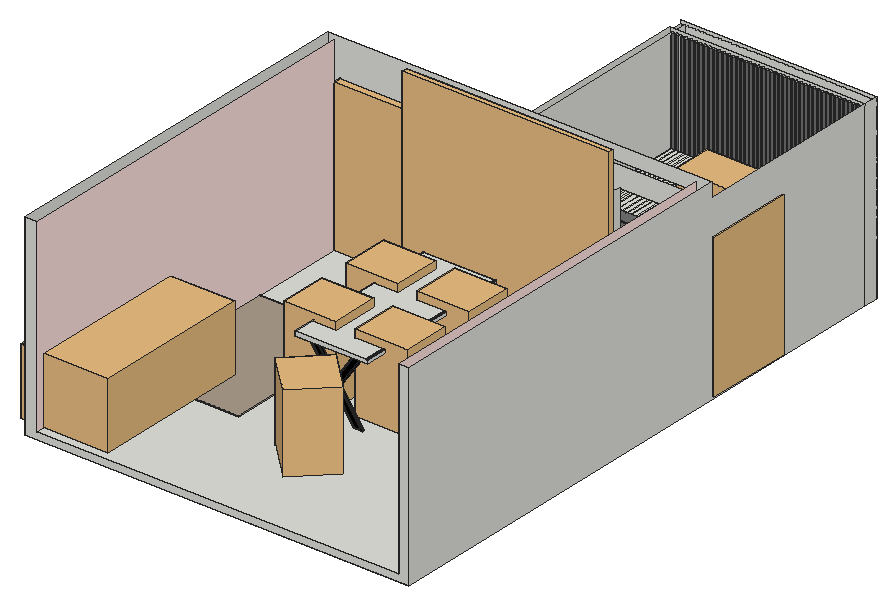
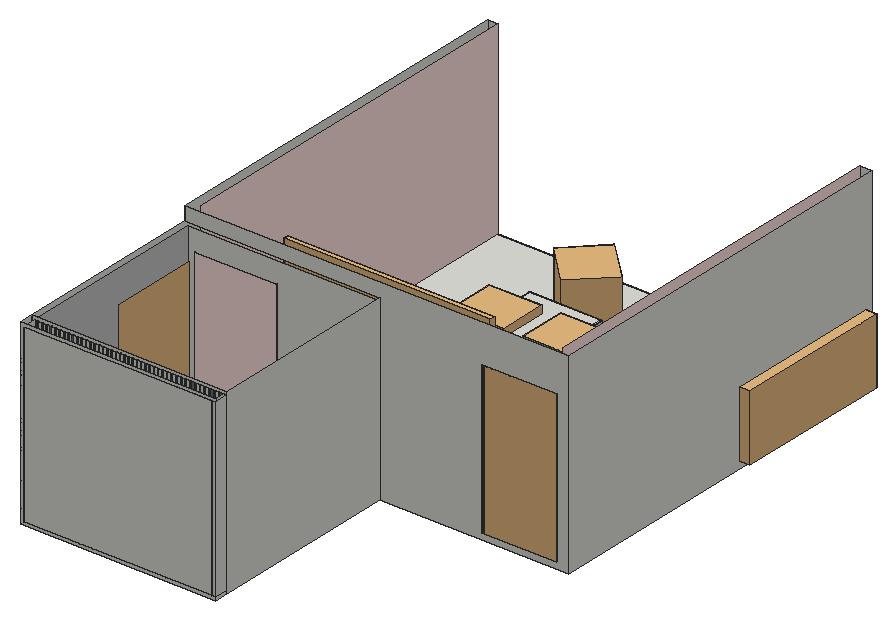
# SketchUp Ruby script. Lengths in inches.
U = 1.inch
M = Sketchup.active_model
def pt(a) = Geom::Point3d.new(a.map { |v| v * U })
def face(e, loops, mat)
  f = e.add_face(loops[0].map { |a| pt(a) })
  loops[1..].each { |l| e.add_face(l.map { |a| pt(a) }).erase! }
  f.material = f.back_material = mat if mat
  f
end
# faces: each face lists its corners as indices into pts; further lists are holes
def faces(e, pts, list, mat = nil) = list.each { |f| face(e, (f[0].is_a?(Array) ? f : [f]).map { |l| l.map { |i| pts[i] } }, mat) }
# xy, xz, yz: faces in a plane at the given z, y or x. An outline is a flat list of corners, or four numbers for a rectangle; further outlines are holes
def ring(l) = l.size == 4 ? [[l[0], l[1]], [l[2], l[1]], [l[2], l[3]], [l[0], l[3]]] : l.each_slice(2).to_a
def flat(e, list, mat, &to3) = list.each { |f| face(e, (f[0].is_a?(Array) ? f : [f]).map { |l| ring(l).map { |u, v| to3.(u, v) } }, mat) }
def xy(e, z, list, mat = nil) = flat(e, list, mat) { |x, y| [x, y, z] }
def xz(e, y, list, mat = nil) = flat(e, list, mat) { |x, z| [x, y, z] }
def yz(e, x, list, mat = nil) = flat(e, list, mat) { |y, z| [x, y, z] }
def lines(e, pts, list) = list.each { |a, b| e.add_line(pt(pts[a]), pt(pts[b])) }
# prism: a flat outline (further loops are holes) pulled along v
def prism(e, loops, v, mat = nil)
  f = face(e, loops, mat); d = Geom::Vector3d.new(v.map { |x| x * U })
  f.pushpull(f.normal.samedirection?(d) ? d.length : -d.length)
end
def box(e, o, s, mat = nil) = prism(e, [[o, [o[0] + s[0], o[1], o[2]], [o[0] + s[0], o[1] + s[1], o[2]], [o[0], o[1] + s[1], o[2]]]], [0, 0, s[2]], mat)
def at(x, y, z, deg = 0) = Geom::Transformation.translation(pt([x, y, z])) * Geom::Transformation.rotation(ORIGIN, Z_AXIS, deg.degrees)
def axes(o, x, y, z) = Geom::Transformation.new([*x, 0, *y, 0, *z, 0, *pt(o).to_a, 1])
def part(name) = M.definitions.add(name)
# library, detail: a bought-in or finely detailed component or shape, given as its bounding box
def library(name, o, s) = part(name).tap { |d| box(d.entities, o, s) }
def detail(e, o, s) = box(e.add_group.entities, o, s)
def put(e, d, t, mat = nil) = e.add_instance(d, t).tap { |i| i.material = mat if mat }
def group(e, t, mat = nil) = e.add_group.tap { |g| g.transformation = t; g.material = mat if mat }.entities
root = M.entities
M.materials.add("[0005_LightPink]").color = [255, 182, 193]
M.materials["[0005_LightPink]"].alpha = 0.48
M.materials.add("[0007_MistyRose]").color = [255, 228, 225]
M.materials.add("[0133_Gray]").color = [128, 128, 128]
M.materials.add("[Color M02]").color = [198, 198, 198]
M.materials.add("[Color M05]").color = [114, 114, 114]
M.materials.add("[Color_009]").color = [0, 0, 0]
M.materials.add("images-82sdfgh").color = [172, 157, 140]
c1 = library("Untitled (23)",[0,0,0],[36,4.39,84])
c2 = library("Agnes+Lisa+(1)",[26.14,-4.33,0],[19.03,22.6,34.8])
c3 = part("Untitled (22)")
g1 = group(c3.entities,at(0,0,0))
box(g1,[0,0,0],[170.08,120.47,0.79],"images-82sdfgh")
c4 = library("Group\#1",[0,0,0],[155.58,4.0625,141.9375])
c5 = part("Group\#5")
xy(c5.entities,0,[[0,0,3.9375,0.79]])
xy(c5.entities,0.39,[[0.74,0,3.73,0.2]])
xy(c5.entities,29.13,[[19.9,0,22.89,0.2]])
xy(c5.entities,29.53,[[19.69,0,23.62,0.79]])
xz(c5.entities,0,[[[0,0,3.9375,0,23.62,29.53,19.69,29.53],[0.74,0.39,19.9,29.13,22.89,29.13,3.73,0.39]]])
xz(c5.entities,0.2,[[0.74,0.39,3.73,0.39,22.89,29.13,19.9,29.13]])
xz(c5.entities,0.79,[[0,0,19.69,29.53,23.62,29.53,3.9375,0]])
p = [[0,0.79,0],[0,0,0],[19.69,0,29.53],[19.69,0.79,29.53],[3.9375,0,0],[3.9375,0.79,0],
  [23.62,0.79,29.53],[23.62,0,29.53],[19.9,0,29.13],[0.74,0,0.39],[0.74,0.2,0.39],[19.9,0.2,29.13],
  [3.73,0,0.39],[22.89,0,29.13],[22.89,0.2,29.13],[3.73,0.2,0.39]]
faces(c5.entities,p,[[0,1,2,3],[4,5,6,7],[8,9,10,11],[12,13,14,15]])
c6 = part("Group\#3")
prism(c6.entities,[[[0.29,0.39,0.77],[0.39,0.39,0.79],[0.5,0.39,0.77],[0.59,0.39,0.73],[0.67,0.39,0.67],[0.73,0.39,0.59],[0.77,0.39,0.5],[0.79,0.39,0.39],[0.77,0.39,0.29],[0.73,0.39,0.2],[0.67,0.39,0.12],[0.59,0.39,0.05],[0.5,0.39,0.01],[0.39,0.39,0],[0.29,0.39,0.01],[0.2,0.39,0.05],[0.12,0.39,0.12],[0.05,0.39,0.2],[0.01,0.39,0.29],[0,0.39,0.39],[0.01,0.39,0.5],[0.05,0.39,0.59],[0.12,0.39,0.67],[0.2,0.39,0.73]]],[0,-0.39,0])
c7 = library("Dahlia+Armchair",[0,-41.1,0],[43.38,78.62,32.87])
c8 = library("Vanity sink assembly",[0,-15.75,0],[23.62,20.08,14.64])
xy(root,0,[[0,0,0,285.5,142.05,285.5,142.05,429.625,289,429.625,289,0],[142.05,429.625,289,440.25]])
xy(root,2.32,[[144.375,285.5,289,285.5,289,351.1875,286.68,351.1875,286.68,428.375,283.99,428.375,283.99,429.625,283.37,429.625,283.37,428.375,280.67,428.375,280.67,429.625,280.05,429.625,280.05,428.375,277.36,428.375,277.36,429.625,276.74,429.625,276.74,428.375,274.05,428.375,274.05,429.625,273.43,429.625,273.43,428.375,270.74,428.375,270.74,429.625,270.12,429.625,270.12,428.375,267.42,428.375,267.42,429.625,266.8,429.625,266.8,428.375,264.11,428.375,264.11,429.625,263.49,429.625,263.49,428.375,260.8,428.375,260.8,429.625,260.18,429.625,260.18,428.375,257.49,428.375,257.49,429.625,256.87,429.625,256.87,428.375,254.17,428.375,254.17,429.625,253.55,429.625,253.55,428.375,250.86,428.375,250.86,429.625,250.24,429.625,250.24,428.375,247.55,428.375,247.55,429.625,247.05,429.625,247.05,428.375,244.36,428.375,244.36,429.625,243.87,429.625,243.87,428.375,241.17,428.375,241.17,429.625,240.68,429.625,240.68,428.375,237.99,428.375,237.99,429.625,237.49,429.625,237.49,428.375,234.8,428.375,234.8,429.625,234.3,429.625,234.3,428.375,231.61,428.375,231.61,429.625,231.12,429.625,231.12,428.375,228.42,428.375,228.42,429.625,227.93,429.625,227.93,428.375,225.24,428.375,225.24,429.625,224.74,429.625,224.74,428.375,222.05,428.375,222.05,429.625,221.55,429.625,221.55,428.375,218.86,428.375,218.86,429.625,218.37,429.625,218.37,428.375,215.67,428.375,215.67,429.625,215.18,429.625,215.18,428.375,212.49,428.375,212.49,429.625,211.99,429.625,211.99,428.375,209.3,428.375,209.3,429.625,208.8,429.625,208.8,428.375,206.11,428.375,206.11,429.625,205.62,429.625,205.62,428.375,202.92,428.375,202.92,429.625,202.43,429.625,202.43,428.375,199.74,428.375,199.74,429.625,199.24,429.625,199.24,428.375,196.55,428.375,196.55,429.625,196.05,429.625,196.05,428.375,193.36,428.375,193.36,429.625,192.87,429.625,192.87,428.375,190.17,428.375,190.17,429.625,189.68,429.625,189.68,428.375,186.99,428.375,186.99,429.625,186.12,429.625,186.12,428.375,183.42,428.375,183.42,429.625,182.55,429.625,182.55,428.375,179.86,428.375,179.86,429.625,178.99,429.625,178.99,428.375,176.3,428.375,176.3,429.625,175.43,429.625,175.43,428.375,172.74,428.375,172.74,429.625,171.87,429.625,171.87,428.375,169.17,428.375,169.17,429.625,168.3,429.625,168.3,428.375,165.61,428.375,165.61,429.625,164.74,429.625,164.74,428.375,162.05,428.375,162.05,429.625,161.18,429.625,161.18,428.375,158.49,428.375,158.49,429.625,157.62,429.625,157.62,428.375,154.92,428.375,154.92,429.625,154.05,429.625,154.05,428.375,151.36,428.375,151.36,429.625,150.49,429.625,150.49,428.375,147.8,428.375,147.8,429.625,146.93,429.625,146.93,428,144.375,428],[144.375,428,146.93,429.625],[147.8,428.375,150.49,429.625],[151.36,428.375,154.05,429.625],[154.92,428.375,157.62,429.625],
  [158.49,428.375,161.18,429.625],[162.05,428.375,164.74,429.625],[165.61,428.375,168.3,429.625],[169.17,428.375,171.87,429.625],[172.74,428.375,175.43,429.625],
  [176.3,428.375,178.99,429.625],[179.86,428.375,182.55,429.625],[183.42,428.375,186.12,429.625],[186.99,428.375,189.68,429.625],[190.17,428.375,192.87,429.625],
  [193.36,428.375,196.05,429.625],[196.55,428.375,199.24,429.625],[199.74,428.375,202.43,429.625],[202.92,428.375,205.62,429.625],[206.11,428.375,208.8,429.625],
  [209.3,428.375,211.99,429.625],[212.49,428.375,215.18,429.625],[215.67,428.375,218.37,429.625],[218.86,428.375,221.55,429.625],[222.05,428.375,224.74,429.625],
  [225.24,428.375,227.93,429.625],[228.42,428.375,231.12,429.625],[231.61,428.375,234.3,429.625],[234.8,428.375,237.49,429.625],[237.99,428.375,240.68,429.625],
  [241.17,428.375,243.87,429.625],[244.36,428.375,247.05,429.625],[247.55,428.375,250.24,429.625],[250.86,428.375,253.55,429.625],[254.17,428.375,256.87,429.625],
  [257.49,428.375,260.18,429.625],[260.8,428.375,263.49,429.625],[264.11,428.375,266.8,429.625],[267.42,428.375,270.12,429.625],[270.74,428.375,273.43,429.625],
  [274.05,428.375,276.74,429.625],[277.36,428.375,280.05,429.625],[280.67,428.375,283.37,429.625],[283.99,428.375,286.68,429.625],[142.05,429.625,144.375,440.25],
  [144.375,429.625,286.68,440.25]])
xy(root,5.0625,[[[8.87,0,281.7,0,281.7,285.5,219.26,285.5,219.26,279.57,63.68,279.57,63.68,285.5,8.87,285.5],[117.04,119.89,118.79,121.76,118.79,119.89]],[117.04,119.89,118.79,119.89,118.79,121.76]])
xy(root,34.75,[[144.375,351.1875,144.375,428,146.93,428,146.93,429.625,147.8,429.625,147.8,428.375,150.49,428.375,150.49,429.625,151.36,429.625,151.36,428.375,154.05,428.375,154.05,429.625,154.92,429.625,154.92,428.375,157.62,428.375,157.62,429.625,158.49,429.625,158.49,428.375,161.18,428.375,161.18,429.625,162.05,429.625,162.05,428.375,164.74,428.375,164.74,429.625,165.61,429.625,165.61,428.375,168.3,428.375,168.3,429.625,169.17,429.625,169.17,428.375,171.87,428.375,171.87,429.625,172.74,429.625,172.74,428.375,175.43,428.375,175.43,429.625,176.3,429.625,176.3,428.375,178.99,428.375,178.99,429.625,179.86,429.625,179.86,428.375,182.55,428.375,182.55,429.625,183.42,429.625,183.42,428.375,186.12,428.375,186.12,429.625,186.99,429.625,186.99,428.375,189.68,428.375,189.68,429.625,190.17,429.625,190.17,428.375,192.87,428.375,192.87,429.625,193.36,429.625,193.36,428.375,196.05,428.375,196.05,429.625,196.55,429.625,196.55,428.375,199.24,428.375,199.24,429.625,199.74,429.625,199.74,428.375,202.43,428.375,202.43,429.625,202.92,429.625,202.92,428.375,205.62,428.375,205.62,429.625,206.11,429.625,206.11,428.375,208.8,428.375,208.8,429.625,209.3,429.625,209.3,428.375,211.99,428.375,211.99,429.625,212.49,429.625,212.49,428.375,215.18,428.375,215.18,429.625,215.67,429.625,215.67,428.375,218.37,428.375,218.37,429.625,218.86,429.625,218.86,428.375,221.55,428.375,221.55,429.625,222.05,429.625,222.05,428.375,224.74,428.375,224.74,429.625,225.24,429.625,225.24,428.375,227.93,428.375,227.93,429.625,228.42,429.625,228.42,428.375,231.12,428.375,231.12,429.625,231.61,429.625,231.61,428.375,234.3,428.375,234.3,429.625,234.8,429.625,234.8,428.375,237.49,428.375,237.49,429.625,237.99,429.625,237.99,428.375,240.68,428.375,240.68,429.625,241.17,429.625,241.17,428.375,243.87,428.375,243.87,429.625,244.36,429.625,244.36,428.375,247.05,428.375,247.05,429.625,247.55,429.625,247.55,428.375,250.24,428.375,250.24,429.625,250.86,429.625,250.86,428.375,253.55,428.375,253.55,429.625,254.17,429.625,254.17,428.375,256.87,428.375,256.87,429.625,257.49,429.625,257.49,428.375,260.18,428.375,260.18,429.625,260.8,429.625,260.8,428.375,263.49,428.375,263.49,429.625,264.11,429.625,264.11,428.375,266.8,428.375,266.8,429.625,267.42,429.625,267.42,428.375,270.12,428.375,270.12,429.625,270.74,429.625,270.74,428.375,273.43,428.375,273.43,429.625,274.05,429.625,274.05,428.375,276.74,428.375,276.74,429.625,277.36,429.625,277.36,428.375,280.05,428.375,280.05,429.625,280.67,429.625,280.67,428.375,283.37,428.375,283.37,429.625,283.99,429.625,283.99,428.375,286.68,428.375,286.68,351.1875]])
xy(root,48.21,[[144.375,351.1875,286.68,353.3125]])
xy(root,49.52,[[144.375,351.1875,286.68,353.3125]])
xy(root,56.41,[[144.375,351.1875,146.93,427.8125],[146.93,351.1875,147.8,429.625],[147.8,351.1875,150.49,427.8125],[150.49,351.1875,151.36,429.625],[151.36,351.1875,154.05,427.8125],
  [154.05,351.1875,154.92,429.625],[154.92,351.1875,157.62,427.8125],[157.62,351.1875,158.49,429.625],[158.49,351.1875,161.18,427.8125],[161.18,351.1875,162.05,429.625],
  [162.05,351.1875,164.74,427.8125],[164.74,351.1875,165.61,429.625],[165.61,351.1875,168.3,427.8125],[168.3,351.1875,169.17,429.625],[169.17,351.1875,171.87,427.8125],
  [171.87,351.1875,172.74,429.625],[172.74,351.1875,175.43,427.8125],[175.43,351.1875,176.3,429.625],[176.3,351.1875,178.99,427.8125],[178.99,351.1875,179.86,429.625],
  [179.86,351.1875,182.55,427.8125],[182.55,351.1875,183.42,429.625],[183.42,351.1875,186.12,427.8125],[186.12,351.1875,186.99,429.625],[186.99,351.1875,189.68,427.8125],
  [189.68,351.1875,190.17,429.625],[190.17,351.1875,192.87,427.8125],[192.87,351.1875,193.36,429.625],[193.36,351.1875,196.05,428.0625],[196.05,351.1875,196.55,429.625],
  [196.55,351.1875,199.24,428.0625],[199.24,351.1875,199.74,429.625],[199.74,351.1875,202.43,428.0625],[202.43,351.1875,202.92,429.625],[202.92,351.1875,205.62,428.0625],
  [205.62,351.1875,206.11,429.625],[206.11,351.1875,208.8,428.0625],[208.8,351.1875,209.3,429.625],[209.3,351.1875,211.99,428.0625],[211.99,351.1875,212.49,429.625],
  [212.49,351.1875,215.18,428.0625],[215.18,351.1875,215.67,429.625],[215.67,351.1875,218.37,428.0625],[218.37,351.1875,218.86,429.625],[218.86,351.1875,221.55,428.0625],
  [221.55,351.1875,222.05,429.625],[222.05,351.1875,224.74,428.0625],[224.74,351.1875,225.24,429.625],[225.24,351.1875,227.93,428.0625],[227.93,351.1875,228.42,429.625],
  [228.42,351.1875,231.12,428.0625],[231.12,351.1875,231.61,429.625],[231.61,351.1875,234.3,428.0625],[234.3,351.1875,234.8,429.625],[234.8,351.1875,237.49,428.0625],
  [237.49,351.1875,237.99,429.625],[237.99,351.1875,240.68,428.0625],[240.68,351.1875,241.17,429.625],[241.17,351.1875,243.87,428.0625],[243.87,351.1875,244.36,429.625],
  [244.36,351.1875,247.05,428.0625],[247.05,351.1875,247.55,429.625],[247.55,351.1875,250.24,428.0625],[250.24,351.1875,250.86,429.625],[250.86,351.1875,253.55,428.375],
  [253.55,351.1875,254.17,429.625],[254.17,351.1875,256.87,428.375],[256.87,351.1875,257.49,429.625],[257.49,351.1875,260.18,428.375],[260.18,351.1875,260.8,429.625],
  [260.8,351.1875,263.49,428.375],[263.49,351.1875,264.11,429.625],[264.11,351.1875,266.8,428.375],[266.8,351.1875,267.42,429.625],[267.42,351.1875,270.12,428.375],
  [270.12,351.1875,270.74,429.625],[270.74,351.1875,273.43,428.375],[273.43,351.1875,274.05,429.625],[274.05,351.1875,276.74,428.375],[276.74,351.1875,277.36,429.625],
  [277.36,351.1875,280.05,428.375],[280.05,351.1875,280.67,429.625],[280.67,351.1875,283.37,428.375],[283.37,351.1875,283.99,429.625],[283.99,351.1875,286.68,428.375]])
xz(root,0,[[0,0,289,0,289,147,281.7,147,281.7,5.0625,8.87,5.0625,8.87,147,0,147]])
xz(root,279.57,[[63.68,5.0625,87.68,5.0625,87.68,147,82.17,147,82.17,146.95,63.68,146.95],[87.68,5.0625,195.26,5.0625,195.26,146.95,88.22,146.95,88.22,147,87.68,147],[195.26,5.0625,219.26,146.95]])
xz(root,285.5,[[[0,0,0,147,289,147,289,136.5,142.05,136.5,142.05,0],[8.87,5.0625,63.68,118.49]],[[144.375,2.32,144.375,134.18,286.68,134.18,286.68,109.95,289,109.95,289,2.32],[219.26,5.0625,281.7,118.74]]])
xz(root,351.1875,[[286.68,2.32,289,109.95]])
xz(root,351.1875,[[144.375,34.75,286.68,48.21],[144.375,49.52,286.68,56.41]],"[0133_Gray]")
xz(root,353.3125,[[144.375,48.21,286.68,49.52]])
xz(root,427.8125,[[144.375,56.41,146.93,134.18],[147.8,56.41,150.49,134.18],[151.36,56.41,154.05,134.18],[154.92,56.41,157.62,134.18],[158.49,56.41,161.18,134.18],
  [162.05,56.41,164.74,134.18],[165.61,56.41,168.3,134.18],[169.17,56.41,171.87,134.18],[172.74,56.41,175.43,134.18],[176.3,56.41,178.99,134.18],
  [179.86,56.41,182.55,134.18],[183.42,56.41,186.12,134.18],[186.99,56.41,189.68,134.18],[190.17,56.41,192.87,134.18]],"[Color M05]")
xz(root,428,[[144.375,2.32,146.93,34.75]],"[Color M05]")
xz(root,428.0625,[[193.36,56.41,196.05,134.18],[196.55,56.41,199.24,134.18],[199.74,56.41,202.43,134.18],[202.92,56.41,205.62,134.18],[206.11,56.41,208.8,134.18],
  [209.3,56.41,211.99,134.18],[212.49,56.41,215.18,134.18],[215.67,56.41,218.37,134.18],[218.86,56.41,221.55,134.18],[222.05,56.41,224.74,134.18],
  [225.24,56.41,227.93,134.18],[228.42,56.41,231.12,134.18],[231.61,56.41,234.3,134.18],[234.8,56.41,237.49,134.18],[237.99,56.41,240.68,134.18],
  [241.17,56.41,243.87,134.18],[244.36,56.41,247.05,134.18],[247.55,56.41,250.24,134.18]],"[Color M05]")
xz(root,428.375,[[147.8,2.32,150.49,34.75],[151.36,2.32,154.05,34.75],[154.92,2.32,157.62,34.75],[158.49,2.32,161.18,34.75],[162.05,2.32,164.74,34.75],
  [165.61,2.32,168.3,34.75],[169.17,2.32,171.87,34.75],[172.74,2.32,175.43,34.75],[176.3,2.32,178.99,34.75],[179.86,2.32,182.55,34.75],
  [183.42,2.32,186.12,34.75],[186.99,2.32,189.68,34.75],[190.17,2.32,192.87,34.75],[193.36,2.32,196.05,34.75],[196.55,2.32,199.24,34.75],
  [199.74,2.32,202.43,34.75],[202.92,2.32,205.62,34.75],[206.11,2.32,208.8,34.75],[209.3,2.32,211.99,34.75],[212.49,2.32,215.18,34.75],
  [215.67,2.32,218.37,34.75],[218.86,2.32,221.55,34.75],[222.05,2.32,224.74,34.75],[225.24,2.32,227.93,34.75],[228.42,2.32,231.12,34.75],
  [231.61,2.32,234.3,34.75],[234.8,2.32,237.49,34.75],[237.99,2.32,240.68,34.75],[241.17,2.32,243.87,34.75],[244.36,2.32,247.05,34.75],
  [247.55,2.32,250.24,34.75],[250.86,2.32,253.55,34.75],[254.17,2.32,256.87,34.75],[257.49,2.32,260.18,34.75],[260.8,2.32,263.49,34.75],
  [264.11,2.32,266.8,34.75],[267.42,2.32,270.12,34.75],[270.74,2.32,273.43,34.75],[274.05,2.32,276.74,34.75],[277.36,2.32,280.05,34.75],
  [280.67,2.32,283.37,34.75],[283.99,2.32,286.68,34.75],[250.86,56.41,253.55,134.18],[254.17,56.41,256.87,134.18],[257.49,56.41,260.18,134.18],
  [260.8,56.41,263.49,134.18],[264.11,56.41,266.8,134.18],[267.42,56.41,270.12,134.18],[270.74,56.41,273.43,134.18],[274.05,56.41,276.74,134.18],
  [277.36,56.41,280.05,134.18],[280.67,56.41,283.37,134.18],[283.99,56.41,286.68,134.18]],"[Color M05]")
xz(root,429.625,[[142.05,0,289,0,289,136.5,142.05,136.5,142.05,134.18,286.68,134.18,286.68,2.32,142.05,2.32],[142.05,2.32,144.24,134.18],[144.24,2.32,144.375,134.18],[189.68,2.32,190.17,34.75],[215.18,56.41,215.67,134.18],
  [227.93,56.41,228.42,134.18]])
xz(root,429.625,[[146.93,2.32,147.8,34.75],[150.49,2.32,151.36,34.75],[154.05,2.32,154.92,34.75],[157.62,2.32,158.49,34.75],[161.18,2.32,162.05,34.75],
  [164.74,2.32,165.61,34.75],[168.3,2.32,169.17,34.75],[171.87,2.32,172.74,34.75],[175.43,2.32,176.3,34.75],[178.99,2.32,179.86,34.75],
  [182.55,2.32,183.42,34.75],[186.12,2.32,186.99,34.75],[192.87,2.32,193.36,34.75],[196.05,2.32,196.55,34.75],[199.24,2.32,199.74,34.75],
  [202.43,2.32,202.92,34.75],[205.62,2.32,206.11,34.75],[208.8,2.32,209.3,34.75],[211.99,2.32,212.49,34.75],[215.18,2.32,215.67,34.75],
  [218.37,2.32,218.86,34.75],[221.55,2.32,222.05,34.75],[224.74,2.32,225.24,34.75],[227.93,2.32,228.42,34.75],[231.12,2.32,231.61,34.75],
  [234.3,2.32,234.8,34.75],[237.49,2.32,237.99,34.75],[240.68,2.32,241.17,34.75],[243.87,2.32,244.36,34.75],[247.05,2.32,247.55,34.75],
  [250.24,2.32,250.86,34.75],[253.55,2.32,254.17,34.75],[256.87,2.32,257.49,34.75],[260.18,2.32,260.8,34.75],[263.49,2.32,264.11,34.75],
  [266.8,2.32,267.42,34.75],[270.12,2.32,270.74,34.75],[273.43,2.32,274.05,34.75],[276.74,2.32,277.36,34.75],[280.05,2.32,280.67,34.75],
  [283.37,2.32,283.99,34.75],[146.93,56.41,147.8,134.18],[150.49,56.41,151.36,134.18],[154.05,56.41,154.92,134.18],[157.62,56.41,158.49,134.18],
  [161.18,56.41,162.05,134.18],[164.74,56.41,165.61,134.18],[168.3,56.41,169.17,134.18],[171.87,56.41,172.74,134.18],[175.43,56.41,176.3,134.18],
  [178.99,56.41,179.86,134.18],[182.55,56.41,183.42,134.18],[186.12,56.41,186.99,134.18],[189.68,56.41,190.17,134.18],[192.87,56.41,193.36,134.18],
  [196.05,56.41,196.55,134.18],[199.24,56.41,199.74,134.18],[202.43,56.41,202.92,134.18],[205.62,56.41,206.11,134.18],[208.8,56.41,209.3,134.18],
  [211.99,56.41,212.49,134.18],[218.37,56.41,218.86,134.18],[221.55,56.41,222.05,134.18],[224.74,56.41,225.24,134.18],[231.12,56.41,231.61,134.18],
  [234.3,56.41,234.8,134.18],[237.49,56.41,237.99,134.18],[240.68,56.41,241.17,134.18],[243.87,56.41,244.36,134.18],[247.05,56.41,247.55,134.18],
  [250.24,56.41,250.86,134.18],[253.55,56.41,254.17,134.18],[256.87,56.41,257.49,134.18],[260.18,56.41,260.8,134.18],[263.49,56.41,264.11,134.18],
  [266.8,56.41,267.42,134.18],[270.12,56.41,270.74,134.18],[273.43,56.41,274.05,134.18],[276.74,56.41,277.36,134.18],[280.05,56.41,280.67,134.18],
  [283.37,56.41,283.99,134.18]],"[Color M05]")
xz(root,440.25,[[142.05,0,142.05,2.32,286.68,2.32,286.68,134.18,142.05,134.18,142.05,136.5,289,136.5,289,0],[142.05,2.32,144.375,134.18],[144.375,2.32,286.68,134.18]])
yz(root,0,[[0,0,285.5,147]])
yz(root,8.87,[[0,5.0625,285.5,5.0625,285.5,118.49,279.57,118.49,279.57,146.95,0,146.95]],"[0007_MistyRose]")
yz(root,63.68,[[279.57,5.0625,285.5,118.49]])
yz(root,142.05,[[285.5,0,429.625,136.5],[429.625,0,440.25,2.32],[429.625,2.32,440.25,134.18]])
yz(root,144.375,[[285.5,2.32,428,2.32,428,34.75,351.1875,34.75,351.1875,48.21,353.3125,48.21,353.3125,49.52,351.1875,49.52,351.1875,56.41,427.8125,56.41,427.8125,134.18,285.5,134.18],[428,2.32,429.625,34.75],[429.625,2.32,440.25,134.18],[351.1875,34.75,429.625,48.21],[353.3125,48.21,429.625,48.21,429.625,56.41,351.1875,56.41,351.1875,49.52,353.3125,49.52],
  [427.8125,56.41,429.625,134.18]])
yz(root,146.93,[[428,2.32,429.625,34.75],[427.8125,56.41,429.625,134.18]],"[Color M05]")
yz(root,147.8,[[428.375,2.32,429.625,34.75],[427.8125,56.41,429.625,134.18]])
yz(root,150.49,[[427.8125,56.41,429.625,134.18]])
yz(root,150.49,[[428.375,2.32,429.625,34.75]],"[Color M05]")
yz(root,151.36,[[428.375,2.32,429.625,34.75],[427.8125,56.41,429.625,134.18]])
yz(root,154.05,[[428.375,2.32,429.625,34.75]])
yz(root,154.05,[[427.8125,56.41,429.625,134.18]],"[Color M05]")
yz(root,154.92,[[428.375,2.32,429.625,34.75],[427.8125,56.41,429.625,134.18]])
yz(root,157.62,[[428.375,2.32,429.625,34.75],[427.8125,56.41,429.625,134.18]])
yz(root,158.49,[[428.375,2.32,429.625,34.75],[427.8125,56.41,429.625,134.18]])
yz(root,161.18,[[428.375,2.32,429.625,34.75],[427.8125,56.41,429.625,134.18]])
yz(root,162.05,[[428.375,2.32,429.625,34.75],[427.8125,56.41,429.625,134.18]])
yz(root,164.74,[[428.375,2.32,429.625,34.75],[427.8125,56.41,429.625,134.18]])
yz(root,165.61,[[428.375,2.32,429.625,34.75],[427.8125,56.41,429.625,134.18]])
yz(root,168.3,[[428.375,2.32,429.625,34.75]])
yz(root,168.3,[[427.8125,56.41,429.625,134.18]],"[Color M05]")
yz(root,169.17,[[428.375,2.32,429.625,34.75],[427.8125,56.41,429.625,134.18]])
yz(root,171.87,[[428.375,2.32,429.625,34.75],[427.8125,56.41,429.625,134.18]])
yz(root,172.74,[[428.375,2.32,429.625,34.75],[427.8125,56.41,429.625,134.18]])
yz(root,175.43,[[428.375,2.32,429.625,34.75],[427.8125,56.41,429.625,134.18]])
yz(root,176.3,[[428.375,2.32,429.625,34.75],[427.8125,56.41,429.625,134.18]])
yz(root,178.99,[[428.375,2.32,429.625,34.75],[427.8125,56.41,429.625,134.18]])
yz(root,179.86,[[428.375,2.32,429.625,34.75]])
yz(root,179.86,[[427.8125,56.41,429.625,134.18]],"[Color M05]")
yz(root,182.55,[[428.375,2.32,429.625,34.75],[427.8125,56.41,429.625,134.18]])
yz(root,183.42,[[428.375,2.32,429.625,34.75],[427.8125,56.41,429.625,134.18]])
yz(root,186.12,[[428.375,2.32,429.625,34.75],[427.8125,56.41,429.625,134.18]])
yz(root,186.99,[[428.375,2.32,429.625,34.75],[427.8125,56.41,429.625,134.18]])
yz(root,189.68,[[428.375,2.32,429.625,34.75],[427.8125,56.41,429.625,134.18]])
yz(root,190.17,[[428.375,2.32,429.625,34.75],[427.8125,56.41,429.625,134.18]])
yz(root,192.87,[[428.375,2.32,429.625,34.75],[427.8125,56.41,429.625,134.18]])
yz(root,193.36,[[428.375,2.32,429.625,34.75],[428.0625,56.41,429.625,134.18]])
yz(root,196.05,[[428.375,2.32,429.625,34.75],[428.0625,56.41,429.625,134.18]])
yz(root,196.55,[[428.375,2.32,429.625,34.75],[428.0625,56.41,429.625,134.18]])
yz(root,199.24,[[428.375,2.32,429.625,34.75],[428.0625,56.41,429.625,134.18]])
yz(root,199.74,[[428.375,2.32,429.625,34.75],[428.0625,56.41,429.625,134.18]])
yz(root,202.43,[[428.375,2.32,429.625,34.75],[428.0625,56.41,429.625,134.18]])
yz(root,202.92,[[428.375,2.32,429.625,34.75],[428.0625,56.41,429.625,134.18]])
yz(root,205.62,[[428.375,2.32,429.625,34.75],[428.0625,56.41,429.625,134.18]])
yz(root,206.11,[[428.375,2.32,429.625,34.75],[428.0625,56.41,429.625,134.18]])
yz(root,208.8,[[428.375,2.32,429.625,34.75],[428.0625,56.41,429.625,134.18]])
yz(root,209.3,[[428.375,2.32,429.625,34.75],[428.0625,56.41,429.625,134.18]])
yz(root,211.99,[[428.0625,56.41,429.625,134.18]])
yz(root,211.99,[[428.375,2.32,429.625,34.75]],"[Color M05]")
yz(root,212.49,[[428.375,2.32,429.625,34.75],[428.0625,56.41,429.625,134.18]])
yz(root,215.18,[[428.375,2.32,429.625,34.75],[428.0625,56.41,429.625,134.18]])
yz(root,215.67,[[428.375,2.32,429.625,34.75],[428.0625,56.41,429.625,134.18]])
yz(root,218.37,[[428.375,2.32,429.625,34.75],[428.0625,56.41,429.625,134.18]])
yz(root,218.86,[[428.375,2.32,429.625,34.75],[428.0625,56.41,429.625,134.18]])
yz(root,219.26,[[279.57,5.0625,285.5,118.74]])
yz(root,221.55,[[428.375,2.32,429.625,34.75],[428.0625,56.41,429.625,134.18]])
yz(root,222.05,[[428.375,2.32,429.625,34.75],[428.0625,56.41,429.625,134.18]])
yz(root,224.74,[[428.375,2.32,429.625,34.75],[428.0625,56.41,429.625,134.18]])
yz(root,225.24,[[428.0625,56.41,429.625,134.18]])
yz(root,225.24,[[428.375,2.32,429.625,34.75]],"[Color M05]")
yz(root,227.93,[[428.375,2.32,429.625,34.75],[428.0625,56.41,429.625,134.18]])
yz(root,228.42,[[428.375,2.32,429.625,34.75],[428.0625,56.41,429.625,134.18]])
yz(root,231.12,[[428.375,2.32,429.625,34.75],[428.0625,56.41,429.625,134.18]])
yz(root,231.61,[[428.375,2.32,429.625,34.75],[428.0625,56.41,429.625,134.18]])
yz(root,234.3,[[428.375,2.32,429.625,34.75],[428.0625,56.41,429.625,134.18]])
yz(root,234.8,[[428.375,2.32,429.625,34.75],[428.0625,56.41,429.625,134.18]])
yz(root,237.49,[[428.375,2.32,429.625,34.75],[428.0625,56.41,429.625,134.18]])
yz(root,237.99,[[428.375,2.32,429.625,34.75],[428.0625,56.41,429.625,134.18]])
yz(root,240.68,[[428.375,2.32,429.625,34.75],[428.0625,56.41,429.625,134.18]])
yz(root,241.17,[[428.375,2.32,429.625,34.75],[428.0625,56.41,429.625,134.18]])
yz(root,243.87,[[428.375,2.32,429.625,34.75],[428.0625,56.41,429.625,134.18]])
yz(root,244.36,[[428.375,2.32,429.625,34.75],[428.0625,56.41,429.625,134.18]])
yz(root,247.05,[[428.375,2.32,429.625,34.75],[428.0625,56.41,429.625,134.18]])
yz(root,247.55,[[428.375,2.32,429.625,34.75],[428.0625,56.41,429.625,134.18]])
yz(root,250.24,[[428.0625,56.41,429.625,134.18]])
yz(root,250.24,[[428.375,2.32,429.625,34.75]],"[Color M05]")
yz(root,250.86,[[428.375,2.32,429.625,34.75],[428.375,56.41,429.625,134.18]])
yz(root,253.55,[[428.375,2.32,429.625,34.75],[428.375,56.41,429.625,134.18]])
yz(root,254.17,[[428.375,2.32,429.625,34.75],[428.375,56.41,429.625,134.18]])
yz(root,256.87,[[428.375,2.32,429.625,34.75],[428.375,56.41,429.625,134.18]])
yz(root,257.49,[[428.375,2.32,429.625,34.75],[428.375,56.41,429.625,134.18]])
yz(root,260.18,[[428.375,2.32,429.625,34.75],[428.375,56.41,429.625,134.18]])
yz(root,260.8,[[428.375,2.32,429.625,34.75],[428.375,56.41,429.625,134.18]])
yz(root,263.49,[[428.375,56.41,429.625,134.18]])
yz(root,263.49,[[428.375,2.32,429.625,34.75]],"[Color M05]")
yz(root,264.11,[[428.375,2.32,429.625,34.75],[428.375,56.41,429.625,134.18]])
yz(root,266.8,[[428.375,2.32,429.625,34.75],[428.375,56.41,429.625,134.18]])
yz(root,267.42,[[428.375,2.32,429.625,34.75],[428.375,56.41,429.625,134.18]])
yz(root,270.12,[[428.375,2.32,429.625,34.75],[428.375,56.41,429.625,134.18]])
yz(root,270.74,[[428.375,2.32,429.625,34.75]])
yz(root,270.74,[[428.375,56.41,429.625,134.18]],"[Color M05]")
yz(root,273.43,[[428.375,2.32,429.625,34.75],[428.375,56.41,429.625,134.18]])
yz(root,274.05,[[428.375,2.32,429.625,34.75]])
yz(root,274.05,[[428.375,56.41,429.625,134.18]],"[Color M05]")
yz(root,276.74,[[428.375,2.32,429.625,34.75],[428.375,56.41,429.625,134.18]])
yz(root,277.36,[[428.375,2.32,429.625,34.75],[428.375,56.41,429.625,134.18]])
yz(root,280.05,[[428.375,2.32,429.625,34.75],[428.375,56.41,429.625,134.18]])
yz(root,280.67,[[428.375,2.32,429.625,34.75],[428.375,56.41,429.625,134.18]])
yz(root,281.7,[[0,5.0625,0,146.95,279.57,146.95,279.57,118.74,285.5,118.74,285.5,5.0625]],"[0007_MistyRose]")
yz(root,283.37,[[428.375,2.32,429.625,34.75],[428.375,56.41,429.625,134.18]])
yz(root,283.99,[[428.375,2.32,429.625,34.75],[428.375,56.41,429.625,134.18]])
yz(root,286.68,[[428.375,2.32,429.625,34.75],[429.625,2.32,440.25,134.18],[351.1875,34.75,429.625,48.21],[351.1875,48.21,353.3125,49.52],[353.3125,48.21,353.3125,49.52,351.1875,49.52,351.1875,56.41,429.625,56.41,429.625,48.21],
  [428.375,56.41,429.625,134.18]])
yz(root,286.68,[[351.1875,2.32,428.375,34.75],[351.1875,56.41,351.1875,109.95,285.5,109.95,285.5,134.18,428.375,134.18,428.375,56.41]],"[Color M02]")
yz(root,289,[[[0,0,429.625,0,429.625,136.5,285.5,136.5,285.5,147,0,147],[285.5,2.32,351.1875,109.95]],[429.625,0,440.25,136.5]])
put(root,c1,axes([286.25,351.1875,2.32],[0,-1.82465,0],[1,0,0],[0,0,1.28125]))
put(root,c2,axes([150.52,216.7,5.0625],[0,-1.87387,0],[1.7427,0,0],[0,0,1.68648]))
put(root,c2,axes([150.52,274.84,5.0625],[0,-1.87387,0],[1.7427,0,0],[0,0,1.68648]))
put(root,c2,axes([121.01,216.7,5.0625],[0,-1.87387,0],[-1.7427,0,0],[0,0,1.68648]))
put(root,c2,axes([121.01,274.84,5.0625],[0,-1.87387,0],[-1.7427,0,0],[0,0,1.68648]))
put(root,c3,axes([0,88.73,5.0625],[0.52821,0,0],[0,1,0],[0,0,1]))
put(root,c1,axes([8.87,279.57,5.0625],[1.55508,0,0],[0,1.37,0],[0,0,1.3503]))
put(root,c4,at(63.68,275.51,5.0625),"[0005_LightPink]")
put(root,c2,axes([192.67,130.6,5.0625],[-1.32503,-1.32503,0],[1.23228,-1.23228,0],[0,0,1.68648]))
g2 = group(root,at(110.18,116.2,5.0625))
put(g2,c5,axes([6.86,5.16,0],[1.7427,0,0],[0,1.87387,0],[0,0,1.68648]),"[Color_009]")
g3 = group(g2,at(48.03,3.6875,0),"[Color_009]")
xy(g3,0,[[-6.86,0,0,1.48]])
xy(g3,0.66,[[-6.49,0,-1.28,0.37]])
xy(g3,49.13,[[-39.88,0,-34.67,0.37]])
xy(g3,49.8,[[-41.17,0,-34.31,1.48]])
xz(g3,0,[[[-6.86,0,-41.17,49.8,-34.31,49.8,0,0],[-6.49,0.66,-1.28,0.66,-34.67,49.13,-39.88,49.13]]])
xz(g3,0.37,[[-6.49,0.66,-39.88,49.13,-34.67,49.13,-1.28,0.66]])
xz(g3,1.48,[[-6.86,0,0,0,-34.31,49.8,-41.17,49.8]])
p = [[-6.86,0,0],[-6.86,1.48,0],[-41.17,1.48,49.8],[-41.17,0,49.8],[0,1.48,0],[0,0,0],
  [-34.31,0,49.8],[-34.31,1.48,49.8],[-6.49,0,0.66],[-39.88,0,49.13],[-39.88,0.37,49.13],[-6.49,0.37,0.66],
  [-34.67,0,49.13],[-1.28,0,0.66],[-1.28,0.37,0.66],[-34.67,0.37,49.13]]
faces(g3,p,[[0,1,2,3],[4,5,6,7],[8,9,10,11],[12,13,14,15]])
put(g2,c5,axes([48.03,115.83,0],[-1.7427,0,0],[0,-1.87387,0],[0,0,1.68648]),"[Color_009]")
put(g2,c6,axes([26.63,3.32,24.27],[1.7427,0,0],[0,1.87387,0],[0,0,1.68648]),"[Color_009]")
put(g2,c6,axes([26.63,116.93,24.27],[1.7427,0,0],[0,1.87387,0],[0,0,1.68648]),"[Color_009]")
put(g2,c5,axes([6.86,117.3,0],[1.7427,0,0],[0,-1.87387,0],[0,0,1.68648]),"[Color_009]")
g4 = group(g2,at(0,3.6875,49.8))
prism(g4,[[[53.86,-3.6875,3.32],[1.03,-3.6875,3.32],[0.76,-3.6875,3.29],[0.51,-3.6875,3.1875],[0.3,-3.6875,3.03],[0.14,-3.6875,2.82],[0.04,-3.6875,2.58],[0,-3.6875,2.32],[0,-3.6875,0],[54.89,-3.6875,0],[54.89,-3.6875,2.32],[54.85,-3.6875,2.58],[54.75,-3.6875,2.82],[54.59,-3.6875,3.03],[54.375,-3.6875,3.1875],[54.125,-3.6875,3.29]]],[0,120.99,0])
put(root,c7,axes([57.74,62.79,5.85],[-1.52,0,0],[0,-1.52,0],[0,0,1.52]))
put(root,c8,axes([184.625,404.96,56.41],[3.50519,0,0],[0,1.49,0],[0,0,1.42235]))
